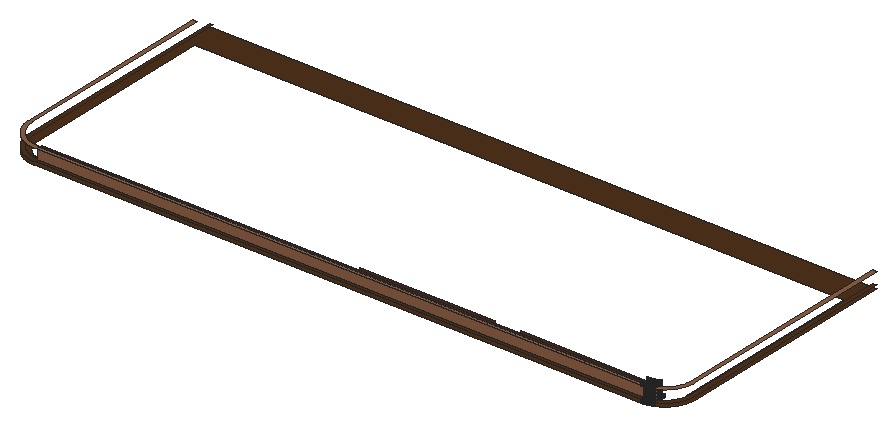
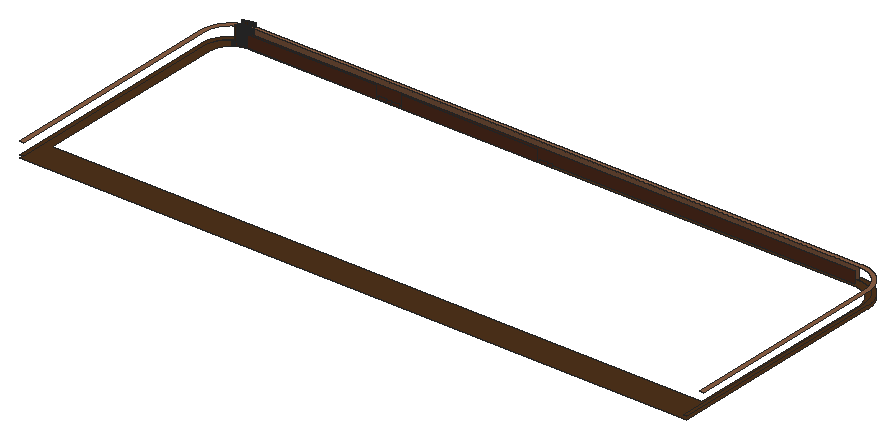
# SketchUp Ruby script. Lengths in inches.
U = 1.inch
M = Sketchup.active_model
def pt(a) = Geom::Point3d.new(a.map { |v| v * U })
def face(e, loops, mat)
  f = e.add_face(loops[0].map { |a| pt(a) })
  loops[1..].each { |l| e.add_face(l.map { |a| pt(a) }).erase! }
  f.material = f.back_material = mat if mat
  f
end
# faces: each face lists its corners as indices into pts; further lists are holes
def faces(e, pts, list, mat = nil) = list.each { |f| face(e, (f[0].is_a?(Array) ? f : [f]).map { |l| l.map { |i| pts[i] } }, mat) }
# xy, xz, yz: faces in a plane at the given z, y or x. An outline is a flat list of corners, or four numbers for a rectangle; further outlines are holes
def ring(l) = l.size == 4 ? [[l[0], l[1]], [l[2], l[1]], [l[2], l[3]], [l[0], l[3]]] : l.each_slice(2).to_a
def flat(e, list, mat, &to3) = list.each { |f| face(e, (f[0].is_a?(Array) ? f : [f]).map { |l| ring(l).map { |u, v| to3.(u, v) } }, mat) }
def xy(e, z, list, mat = nil) = flat(e, list, mat) { |x, y| [x, y, z] }
def xz(e, y, list, mat = nil) = flat(e, list, mat) { |x, z| [x, y, z] }
def yz(e, x, list, mat = nil) = flat(e, list, mat) { |y, z| [x, y, z] }
def lines(e, pts, list) = list.each { |a, b| e.add_line(pt(pts[a]), pt(pts[b])) }
# prism: a flat outline (further loops are holes) pulled along v
def prism(e, loops, v, mat = nil)
  f = face(e, loops, mat); d = Geom::Vector3d.new(v.map { |x| x * U })
  f.pushpull(f.normal.samedirection?(d) ? d.length : -d.length)
end
def box(e, o, s, mat = nil) = prism(e, [[o, [o[0] + s[0], o[1], o[2]], [o[0] + s[0], o[1] + s[1], o[2]], [o[0], o[1] + s[1], o[2]]]], [0, 0, s[2]], mat)
def at(x, y, z, deg = 0) = Geom::Transformation.translation(pt([x, y, z])) * Geom::Transformation.rotation(ORIGIN, Z_AXIS, deg.degrees)
def axes(o, x, y, z) = Geom::Transformation.new([*x, 0, *y, 0, *z, 0, *pt(o).to_a, 1])
def part(name) = M.definitions.add(name)
# library, detail: a bought-in or finely detailed component or shape, given as its bounding box
def library(name, o, s) = part(name).tap { |d| box(d.entities, o, s) }
def detail(e, o, s) = box(e.add_group.entities, o, s)
def put(e, d, t, mat = nil) = e.add_instance(d, t).tap { |i| i.material = mat if mat }
def group(e, t, mat = nil) = e.add_group.tap { |g| g.transformation = t; g.material = mat if mat }.entities
root = M.entities
M.materials.add("1799 AP 8574 BURNISHED CARAMEL").color = [140, 96, 69]
M.materials.add("1816 AP K197 Dark Kaapi-N").color = [79, 50, 27]
M.materials.add("[Wood Cherry Original]1").color = [93, 50, 33]
xy(root,390,[[[65.76,78,65.53,78.01,65.29,78.01,65.06,78.02,64.82,78.04,64.59,78.06,64.35,78.08,64.12,78.1,63.88,78.125,63.65,78.15,63.42,78.1875,63.18,78.22,62.72,78.3,62.49,78.35,62.26,78.39,62.03,78.44,61.8,78.5,61.57,78.55,61.34,78.61,61.11,78.68,60.89,78.74,60.66,78.81,60.4375,78.88,60.21,78.96,59.99,79.03,59.77,79.11,59.55,79.2,59.33,79.28,58.89,79.46,58.68,79.56,58.46,79.65,58.25,79.75,58.04,79.86,57.83,79.96,57.41,80.18,57.2,80.3,57,80.41,56.6,80.65,56.39,80.78,56.2,80.9,56,81.03,55.8,81.17,55.61,81.3,55.42,81.4375,55.23,81.58,55.04,81.72,54.86,81.86,54.67,82.01,54.49,82.16,54.31,82.3125,54.13,82.47,53.96,82.625,53.78,82.78,53.61,82.94,53.44,83.11,53.27,83.27,53.11,83.44,52.94,83.61,52.78,83.78,52.625,83.96,52.47,84.13,52.3125,84.31,52.16,84.49,52.01,84.67,51.86,84.86,51.72,85.04,51.58,85.23,51.4375,85.42,51.3,85.61,51.17,85.8,51.03,86,50.9,86.2,50.78,86.39,50.65,86.6,50.41,87,50.3,87.2,50.18,87.41,49.96,87.83,49.86,88.04,49.75,88.25,49.65,88.46,49.56,88.68,49.46,88.89,49.28,89.33,49.2,89.55,49.11,89.77,49.03,89.99,48.96,90.21,48.88,90.4375,48.81,90.66,48.74,90.89,48.68,91.11,48.61,91.34,48.55,91.57,48.5,91.8,48.44,92.03,48.39,92.26,48.35,92.49,48.3,92.72,48.22,93.18,48.1875,93.42,48.15,93.65,48.125,93.88,48.1,94.12,48.08,94.35,48.06,94.59,48.04,94.82,48.02,95.06,48.01,95.29,48.01,95.53,48,95.76,48,228,438,228,438,95.76,437.99,95.53,437.99,95.29,437.98,95.06,437.96,94.82,437.94,94.59,437.92,94.35,437.9,94.12,437.875,93.88,437.85,93.65,437.8125,93.42,437.78,93.18,437.7,92.72,437.65,92.49,437.61,92.26,437.56,92.03,437.5,91.8,437.45,91.57,437.39,91.34,437.32,91.11,437.26,90.89,437.19,90.66,437.12,90.4375,437.04,90.21,436.97,89.99,436.89,89.77,436.8,89.55,436.72,89.33,436.54,88.89,436.44,88.68,436.35,88.46,436.25,88.25,436.14,88.04,436.04,87.83,435.82,87.41,435.7,87.2,435.59,87,435.35,86.6,435.22,86.39,435.1,86.2,434.97,86,434.83,85.8,434.7,85.61,434.5625,85.42,434.42,85.23,434.28,85.04,434.14,84.86,433.99,84.67,433.84,84.49,433.6875,84.31,433.53,84.13,433.375,83.96,433.22,83.78,433.06,83.61,432.89,83.44,432.73,83.27,432.56,83.11,432.39,82.94,432.22,82.78,432.04,82.625,431.87,82.47,431.69,82.3125,431.51,82.16,431.33,82.01,431.14,81.86,430.96,81.72,430.77,81.58,430.58,81.4375,430.39,81.3,430.2,81.17,430,81.03,429.8,80.9,429.61,80.78,429.4,80.65,429,80.41,428.8,80.3,428.59,80.18,428.17,79.96,427.96,79.86,427.75,79.75,427.54,79.65,427.32,79.56,427.11,79.46,426.67,79.28,426.45,79.2,426.23,79.11,426.01,79.03,425.79,78.96,425.5625,78.88,425.34,78.81,425.11,78.74,424.89,78.68,424.66,78.61,424.43,78.55,424.2,78.5,423.97,78.44,423.74,78.39,423.51,78.35,423.28,78.3,422.82,78.22,422.58,78.1875,422.35,78.15,422.12,78.125,421.88,78.1,421.65,78.08,421.41,78.06,421.18,78.04,420.94,78.02,420.71,78.01,420.47,78.01,420.24,78],[65.66,83,420.34,83,421.19,83.05,421.87,83.13,422.03,83.16,422.2,83.1875,422.37,83.22,422.54,83.25,422.7,83.28,422.87,83.32,423.03,83.36,423.2,83.4,423.36,83.44,423.53,83.49,423.69,83.54,423.86,83.58,424.02,83.64,424.18,83.69,424.34,83.75,424.5,83.8,424.66,83.86,424.82,83.93,424.97,83.99,425.13,84.06,425.29,84.125,425.44,84.19,425.6,84.27,425.75,84.34,426.5,84.74,426.65,84.83,426.79,84.92,426.9375,85.01,427.08,85.1,427.22,85.19,427.36,85.29,427.5,85.38,427.78,85.58,427.91,85.6875,428.05,85.79,428.18,85.9,428.3125,86.01,428.44,86.11,428.57,86.23,428.7,86.34,428.82,86.45,428.95,86.57,429.07,86.6875,429.19,86.81,429.3125,86.93,429.43,87.05,429.55,87.18,429.66,87.3,429.77,87.43,429.89,87.56,429.99,87.6875,430.1,87.82,430.21,87.95,430.3125,88.09,430.42,88.22,430.62,88.5,430.71,88.64,430.81,88.78,430.9,88.92,430.99,89.0625,431.08,89.21,431.17,89.35,431.26,89.5,431.66,90.25,431.73,90.4,431.81,90.56,431.875,90.71,431.94,90.87,432.01,91.03,432.07,91.18,432.14,91.34,432.2,91.5,432.25,91.66,432.31,91.82,432.36,91.98,432.42,92.14,432.46,92.31,432.51,92.47,432.56,92.64,432.6,92.8,432.64,92.97,432.68,93.13,432.72,93.3,432.75,93.46,432.78,93.63,432.8125,93.8,432.84,93.97,432.87,94.13,432.95,94.81,433,95.66,433,211,53,211,53,95.66,53.05,94.81,53.13,94.13,53.16,93.97,53.1875,93.8,53.22,93.63,53.25,93.46,53.28,93.3,53.32,93.13,53.36,92.97,53.4,92.8,53.44,92.64,53.49,92.47,53.54,92.31,53.58,92.14,53.64,91.98,53.69,91.82,53.75,91.66,53.8,91.5,53.86,91.34,53.93,91.18,53.99,91.03,54.06,90.87,54.125,90.71,54.19,90.56,54.27,90.4,54.34,90.25,54.74,89.5,54.83,89.35,54.92,89.21,55.01,89.0625,55.1,88.92,55.19,88.78,55.29,88.64,55.38,88.5,55.58,88.22,55.6875,88.09,55.79,87.95,55.9,87.82,56.01,87.6875,56.11,87.56,56.23,87.43,56.34,87.3,56.45,87.18,56.57,87.05,56.6875,86.93,56.81,86.81,56.93,86.6875,57.05,86.57,57.18,86.45,57.3,86.34,57.43,86.23,57.56,86.11,57.6875,86.01,57.82,85.9,57.95,85.79,58.09,85.6875,58.22,85.58,58.5,85.38,58.64,85.29,58.78,85.19,58.92,85.1,59.0625,85.01,59.21,84.92,59.35,84.83,59.5,84.74,60.25,84.34,60.4,84.27,60.56,84.19,60.71,84.125,60.87,84.06,61.03,83.99,61.18,83.93,61.34,83.86,61.5,83.8,61.66,83.75,61.82,83.69,61.98,83.64,62.14,83.58,62.31,83.54,62.47,83.49,62.64,83.44,62.8,83.4,62.97,83.36,63.13,83.32,63.3,83.28,63.46,83.25,63.63,83.22,63.8,83.1875,63.97,83.16,64.13,83.13,64.81,83.05]]],"1816 AP K197 Dark Kaapi-N")
xy(root,391,[[421.5,84.6,421.92,84.66,421.8,84.64],[421.92,84.66,422.37,84.75,422.8,84.85,423.24,84.97,423.67,85.11,424.09,85.26,424.51,85.43,424.92,85.61,425.32,85.81,425.48,85.9,425.48,85.89,425.35,85.82,425.09,85.6875,424.95,85.62,424.68,85.49,424.4,85.375,423.98,85.21,423.7,85.11,423.12,84.93,422.83,84.85,422.54,84.78,422.24,84.72,422.1,84.69]],"[Wood Cherry Original]1")
xy(root,392,[[65.76,78,420.24,78,420.47,78.01,420.71,78.01,420.94,78.02,421.18,78.04,421.41,78.06,421.65,78.08,421.88,78.1,422.12,78.125,422.35,78.15,422.58,78.1875,422.82,78.22,423.28,78.3,423.51,78.35,423.74,78.39,423.97,78.44,424.2,78.5,424.43,78.55,424.66,78.61,424.89,78.68,425.11,78.74,425.34,78.81,425.5625,78.88,425.79,78.96,426.01,79.03,426.23,79.11,426.45,79.2,426.67,79.28,427.11,79.46,427.32,79.56,427.54,79.65,427.75,79.75,427.96,79.86,428.17,79.96,428.59,80.18,428.8,80.3,429,80.41,429.4,80.65,429.61,80.78,429.8,80.9,430,81.03,430.2,81.17,430.39,81.3,430.58,81.4375,430.77,81.58,430.96,81.72,431.14,81.86,431.33,82.01,431.51,82.16,431.69,82.3125,431.87,82.47,432.04,82.625,432.22,82.78,432.39,82.94,432.56,83.11,432.73,83.27,432.89,83.44,433.06,83.61,433.22,83.78,433.375,83.96,433.53,84.13,433.6875,84.31,433.84,84.49,433.99,84.67,434.14,84.86,434.28,85.04,434.42,85.23,434.5625,85.42,434.7,85.61,434.83,85.8,434.97,86,435.1,86.2,435.22,86.39,435.35,86.6,435.59,87,435.7,87.2,435.82,87.41,436.04,87.83,436.14,88.04,436.25,88.25,436.35,88.46,436.44,88.68,436.54,88.89,436.72,89.33,436.8,89.55,436.89,89.77,436.97,89.99,437.04,90.21,437.12,90.4375,437.19,90.66,437.26,90.89,437.32,91.11,437.39,91.34,437.45,91.57,437.5,91.8,437.56,92.03,437.61,92.26,437.65,92.49,437.7,92.72,437.78,93.18,437.8125,93.42,437.85,93.65,437.875,93.88,437.9,94.12,437.92,94.35,437.94,94.59,437.96,94.82,437.98,95.06,437.99,95.29,437.99,95.53,438,95.76,438,228,436,228,436,95.79,435.99,95.58,435.99,95.37,435.97,94.95,435.95,94.74,435.93,94.54,435.89,94.12,435.83,93.7,435.8,93.5,435.77,93.29,435.73,93.08,435.69,92.88,435.65,92.67,435.61,92.47,435.56,92.26,435.51,92.0625,435.45,91.86,435.4,91.66,435.22,91.06,435.01,90.46,434.9375,90.27,434.86,90.07,434.78,89.88,434.7,89.68,434.62,89.49,434.35,88.92,434.26,88.74,434.16,88.55,434.0625,88.37,433.96,88.18,433.86,88,433.53,87.46,433.42,87.29,433.3,87.11,433.1875,86.9375,433.07,86.77,432.94,86.6,432.82,86.43,432.69,86.26,432.57,86.09,432.43,85.93,432.17,85.61,431.89,85.29,431.61,84.99,431.46,84.84,431.3125,84.6875,431.16,84.54,431.01,84.39,430.71,84.11,430.39,83.83,430.07,83.57,429.91,83.43,429.74,83.31,429.57,83.18,429.4,83.06,429.23,82.93,429.0625,82.8125,428.89,82.7,428.71,82.58,428.54,82.47,428,82.14,427.82,82.04,427.63,81.9375,427.45,81.84,427.26,81.74,427.08,81.65,426.51,81.38,426.32,81.3,426.12,81.22,425.93,81.14,425.73,81.0625,425.54,80.99,424.94,80.78,424.34,80.6,424.14,80.55,423.9375,80.49,423.74,80.44,423.53,80.39,423.33,80.35,423.12,80.31,422.92,80.27,422.71,80.23,422.5,80.2,422.3,80.17,421.88,80.11,421.46,80.07,421.26,80.05,421.05,80.03,420.63,80.01,420.42,80.01,420.21,80,65.79,80,65.58,80.01,65.37,80.01,64.95,80.03,64.74,80.05,64.54,80.07,64.12,80.11,63.7,80.17,63.5,80.2,63.29,80.23,63.08,80.27,62.88,80.31,62.67,80.35,62.47,80.39,62.26,80.44,62.0625,80.49,61.86,80.55,61.66,80.6,61.06,80.78,60.46,80.99,60.27,81.0625,60.07,81.14,59.88,81.22,59.68,81.3,59.49,81.38,58.92,81.65,58.74,81.74,58.55,81.84,58.37,81.9375,58.18,82.04,58,82.14,57.46,82.47,57.29,82.58,57.11,82.7,56.9375,82.8125,56.77,82.93,56.6,83.06,56.43,83.18,56.26,83.31,56.09,83.43,55.93,83.57,55.61,83.83,55.29,84.11,54.99,84.39,54.84,84.54,54.6875,84.6875,54.54,84.84,54.39,84.99,54.11,85.29,53.83,85.61,53.57,85.93,53.43,86.09,53.31,86.26,53.18,86.43,53.06,86.6,52.93,86.77,52.8125,86.9375,52.7,87.11,52.58,87.29,52.47,87.46,52.14,88,52.04,88.18,51.9375,88.37,51.84,88.55,51.74,88.74,51.65,88.92,51.38,89.49,51.3,89.68,51.22,89.88,51.14,90.07,51.0625,90.27,50.99,90.46,50.78,91.06,50.6,91.66,50.55,91.86,50.49,92.0625,50.44,92.26,50.39,92.47,50.35,92.67,50.31,92.88,50.27,93.08,50.23,93.29,50.2,93.5,50.17,93.7,50.11,94.12,50.07,94.54,50.05,94.74,50.03,94.95,50.01,95.37,50.01,95.58,50,95.79,50,228,48,228,48,95.76,48.01,95.53,48.01,95.29,48.02,95.06,48.04,94.82,48.06,94.59,48.08,94.35,48.1,94.12,48.125,93.88,48.15,93.65,48.1875,93.42,48.22,93.18,48.3,92.72,48.35,92.49,48.39,92.26,48.44,92.03,48.5,91.8,48.55,91.57,48.61,91.34,48.68,91.11,48.74,90.89,48.81,90.66,48.88,90.4375,48.96,90.21,49.03,89.99,49.11,89.77,49.2,89.55,49.28,89.33,49.46,88.89,49.56,88.68,49.65,88.46,49.75,88.25,49.86,88.04,49.96,87.83,50.18,87.41,50.3,87.2,50.41,87,50.65,86.6,50.78,86.39,50.9,86.2,51.03,86,51.17,85.8,51.3,85.61,51.4375,85.42,51.58,85.23,51.72,85.04,51.86,84.86,52.01,84.67,52.16,84.49,52.3125,84.31,52.47,84.13,52.625,83.96,52.78,83.78,52.94,83.61,53.11,83.44,53.27,83.27,53.44,83.11,53.61,82.94,53.78,82.78,53.96,82.625,54.13,82.47,54.31,82.3125,54.49,82.16,54.67,82.01,54.86,81.86,55.04,81.72,55.23,81.58,55.42,81.4375,55.61,81.3,55.8,81.17,56,81.03,56.2,80.9,56.39,80.78,56.6,80.65,57,80.41,57.2,80.3,57.41,80.18,57.83,79.96,58.04,79.86,58.25,79.75,58.46,79.65,58.68,79.56,58.89,79.46,59.33,79.28,59.55,79.2,59.77,79.11,59.99,79.03,60.21,78.96,60.4375,78.88,60.66,78.81,60.89,78.74,61.11,78.68,61.34,78.61,61.57,78.55,61.8,78.5,62.03,78.44,62.26,78.39,62.49,78.35,62.72,78.3,63.18,78.22,63.42,78.1875,63.65,78.15,63.88,78.125,64.12,78.1,64.35,78.08,64.59,78.06,64.82,78.04,65.06,78.02,65.29,78.01,65.53,78.01]],"1816 AP K197 Dark Kaapi-N")
xy(root,399,[[65.76,78,65.53,78.01,65.29,78.01,65.06,78.02,64.82,78.04,64.59,78.06,64.35,78.08,64.12,78.1,63.88,78.125,63.65,78.15,63.42,78.1875,63.18,78.22,62.72,78.3,62.49,78.35,62.26,78.39,62.03,78.44,61.8,78.5,61.57,78.55,61.34,78.61,61.11,78.68,60.89,78.74,60.66,78.81,60.4375,78.88,60.21,78.96,59.99,79.03,59.77,79.11,59.55,79.2,59.33,79.28,58.89,79.46,58.68,79.56,58.46,79.65,58.25,79.75,58.04,79.86,57.83,79.96,57.41,80.18,57.2,80.3,57,80.41,56.6,80.65,56.39,80.78,56.2,80.9,56,81.03,55.8,81.17,55.61,81.3,55.42,81.4375,55.23,81.58,55.04,81.72,54.86,81.86,54.67,82.01,54.49,82.16,54.31,82.3125,54.13,82.47,53.96,82.625,53.78,82.78,53.61,82.94,53.44,83.11,53.27,83.27,53.11,83.44,52.94,83.61,52.78,83.78,52.625,83.96,52.47,84.13,52.3125,84.31,52.16,84.49,52.01,84.67,51.86,84.86,51.72,85.04,51.58,85.23,51.4375,85.42,51.3,85.61,51.17,85.8,51.03,86,50.9,86.2,50.78,86.39,50.65,86.6,50.41,87,50.3,87.2,50.18,87.41,49.96,87.83,49.86,88.04,49.75,88.25,49.65,88.46,49.56,88.68,49.46,88.89,49.28,89.33,49.2,89.55,49.11,89.77,49.03,89.99,48.96,90.21,48.88,90.4375,48.81,90.66,48.74,90.89,48.68,91.11,48.61,91.34,48.55,91.57,48.5,91.8,48.44,92.03,48.39,92.26,48.35,92.49,48.3,92.72,48.22,93.18,48.1875,93.42,48.15,93.65,48.125,93.88,48.1,94.12,48.08,94.35,48.06,94.59,48.04,94.82,48.02,95.06,48.01,95.29,48.01,95.53,48,95.76,48,216,50,216,50,95.79,50.01,95.58,50.01,95.37,50.03,94.95,50.05,94.74,50.07,94.54,50.11,94.12,50.17,93.7,50.2,93.5,50.23,93.29,50.27,93.08,50.31,92.88,50.35,92.67,50.39,92.47,50.44,92.26,50.49,92.0625,50.55,91.86,50.6,91.66,50.78,91.06,50.99,90.46,51.0625,90.27,51.14,90.07,51.22,89.88,51.3,89.68,51.38,89.49,51.65,88.92,51.74,88.74,51.84,88.55,51.9375,88.37,52.04,88.18,52.14,88,52.47,87.46,52.58,87.29,52.7,87.11,52.8125,86.9375,52.93,86.77,53.06,86.6,53.18,86.43,53.31,86.26,53.43,86.09,53.57,85.93,53.83,85.61,54.11,85.29,54.39,84.99,54.54,84.84,54.6875,84.6875,54.84,84.54,54.99,84.39,55.29,84.11,55.61,83.83,55.93,83.57,56.09,83.43,56.26,83.31,56.43,83.18,56.6,83.06,56.77,82.93,56.9375,82.8125,57.11,82.7,57.29,82.58,57.46,82.47,58,82.14,58.18,82.04,58.37,81.9375,58.55,81.84,58.74,81.74,58.92,81.65,59.49,81.38,59.68,81.3,59.88,81.22,60.07,81.14,60.27,81.0625,60.46,80.99,61.06,80.78,61.66,80.6,61.86,80.55,62.0625,80.49,62.26,80.44,62.47,80.39,62.67,80.35,62.88,80.31,63.08,80.27,63.29,80.23,63.5,80.2,63.7,80.17,64.12,80.11,64.54,80.07,64.74,80.05,64.95,80.03,65.37,80.01,65.58,80.01,65.79,80,420.21,80,420.42,80.01,420.63,80.01,421.05,80.03,421.26,80.05,421.46,80.07,421.88,80.11,422.3,80.17,422.5,80.2,422.71,80.23,422.92,80.27,423.12,80.31,423.33,80.35,423.53,80.39,423.74,80.44,423.9375,80.49,424.14,80.55,424.34,80.6,424.94,80.78,425.54,80.99,425.73,81.0625,425.93,81.14,426.12,81.22,426.32,81.3,426.51,81.38,427.08,81.65,427.26,81.74,427.45,81.84,427.63,81.9375,427.82,82.04,428,82.14,428.54,82.47,428.71,82.58,428.89,82.7,429.0625,82.8125,429.23,82.93,429.4,83.06,429.57,83.18,429.74,83.31,429.91,83.43,430.07,83.57,430.39,83.83,430.71,84.11,431.01,84.39,431.16,84.54,431.3125,84.6875,431.46,84.84,431.61,84.99,431.89,85.29,432.17,85.61,432.43,85.93,432.57,86.09,432.69,86.26,432.82,86.43,432.94,86.6,433.07,86.77,433.1875,86.9375,433.3,87.11,433.42,87.29,433.53,87.46,433.86,88,433.96,88.18,434.0625,88.37,434.16,88.55,434.26,88.74,434.35,88.92,434.62,89.49,434.7,89.68,434.78,89.88,434.86,90.07,434.9375,90.27,435.01,90.46,435.22,91.06,435.4,91.66,435.45,91.86,435.51,92.0625,435.56,92.26,435.61,92.47,435.65,92.67,435.69,92.88,435.73,93.08,435.77,93.29,435.8,93.5,435.83,93.7,435.89,94.12,435.93,94.54,435.95,94.74,435.97,94.95,435.99,95.37,435.99,95.58,436,95.79,436,228,438,228,438,95.76,437.99,95.53,437.99,95.29,437.98,95.06,437.96,94.82,437.94,94.59,437.92,94.35,437.9,94.12,437.875,93.88,437.85,93.65,437.8125,93.42,437.78,93.18,437.7,92.72,437.65,92.49,437.61,92.26,437.56,92.03,437.5,91.8,437.45,91.57,437.39,91.34,437.32,91.11,437.26,90.89,437.19,90.66,437.12,90.4375,437.04,90.21,436.97,89.99,436.89,89.77,436.8,89.55,436.72,89.33,436.54,88.89,436.44,88.68,436.35,88.46,436.25,88.25,436.14,88.04,436.04,87.83,435.82,87.41,435.7,87.2,435.59,87,435.35,86.6,435.22,86.39,435.1,86.2,434.97,86,434.83,85.8,434.7,85.61,434.5625,85.42,434.42,85.23,434.28,85.04,434.14,84.86,433.99,84.67,433.84,84.49,433.6875,84.31,433.53,84.13,433.375,83.96,433.22,83.78,433.06,83.61,432.89,83.44,432.73,83.27,432.56,83.11,432.39,82.94,432.22,82.78,432.04,82.625,431.87,82.47,431.69,82.3125,431.51,82.16,431.33,82.01,431.14,81.86,430.96,81.72,430.77,81.58,430.58,81.4375,430.39,81.3,430.2,81.17,430,81.03,429.8,80.9,429.61,80.78,429.4,80.65,429,80.41,428.8,80.3,428.59,80.18,428.17,79.96,427.96,79.86,427.75,79.75,427.54,79.65,427.32,79.56,427.11,79.46,426.67,79.28,426.45,79.2,426.23,79.11,426.01,79.03,425.79,78.96,425.5625,78.88,425.34,78.81,425.11,78.74,424.89,78.68,424.66,78.61,424.43,78.55,424.2,78.5,423.97,78.44,423.74,78.39,423.51,78.35,423.28,78.3,422.82,78.22,422.58,78.1875,422.35,78.15,422.12,78.125,421.88,78.1,421.65,78.08,421.41,78.06,421.18,78.04,420.94,78.02,420.71,78.01,420.47,78.01,420.24,78]],"1799 AP 8574 BURNISHED CARAMEL")
xz(root,78,[[420,390,420.24,392],[420,399,420.24,401]],"1816 AP K197 Dark Kaapi-N")
xz(root,78.01,[[420.47,390,420.71,392],[420.47,399,420.71,401]],"1816 AP K197 Dark Kaapi-N")
xz(root,80,[[66.01,392,419.99,399],[419.99,392,420.21,399]],"1799 AP 8574 BURNISHED CARAMEL")
xz(root,80.01,[[420.42,392,420.63,399]],"1799 AP 8574 BURNISHED CARAMEL")
xz(root,83,[[419.98,390,420.17,401],[420.17,390,420.34,401]],"1816 AP K197 Dark Kaapi-N")
xz(root,83,[[66.02,391,419.98,398],[419.98,391,420.17,398],[420.17,391,420.34,398]],"[Wood Cherry Original]1")
xz(root,84.5,[[242,391,244,392.75],[245,391,249,392.75],[250.5,391,329.75,398],[331.25,391,335.25,392.75],[336.25,391,338.25,392.75],
  [339.25,391,343.25,392.75],[344.75,391,419.98,398]],"[Wood Cherry Original]1")
xz(root,84.6,[[421.48,391,421.5,392.75]],"[Wood Cherry Original]1")
p = [[420.24,78,390],[420.47,78.01,390],[420.47,78.01,392],[420.24,78,392],[420.71,78.01,390],[420.94,78.02,390],
  [420.94,78.02,392],[420.71,78.01,392],[421.18,78.04,390],[421.18,78.04,392],[421.41,78.06,390],[421.41,78.06,392],
  [421.65,78.08,390],[421.65,78.08,392],[421.88,78.1,390],[421.88,78.1,392],[422.12,78.125,390],[422.12,78.125,392],
  [422.35,78.15,390],[422.35,78.15,392],[422.58,78.1875,390],[422.58,78.1875,392],[422.82,78.22,390],[422.82,78.22,392],
  [423.05,78.26,390],[423.05,78.26,392],[423.28,78.3,390],[423.28,78.3,392],[423.51,78.35,390],[423.51,78.35,392],
  [423.74,78.39,390],[423.74,78.39,392],[423.97,78.44,390],[423.97,78.44,392],[424.2,78.5,390],[424.2,78.5,392],
  [424.43,78.55,390],[424.43,78.55,392],[424.66,78.61,390],[424.66,78.61,392],[424.89,78.68,390],[424.89,78.68,392],
  [425.11,78.74,390],[425.11,78.74,392],[425.34,78.81,390],[425.34,78.81,392],[425.5625,78.88,390],[425.5625,78.88,392],
  [425.79,78.96,390],[425.79,78.96,392],[426.01,79.03,390],[426.01,79.03,392],[426.23,79.11,390],[426.23,79.11,392],
  [426.45,79.2,390],[426.45,79.2,392],[426.67,79.28,390],[426.67,79.28,392],[426.89,79.37,390],[426.89,79.37,392],
  [427.11,79.46,390],[427.11,79.46,392],[420.34,83,401],[420.51,83.01,401],[420.51,83.01,390],[420.34,83,390],
  [420.68,83.02,401],[420.68,83.02,390],[420.85,83.03,401],[420.85,83.03,390],[421.02,83.04,401],[421.02,83.04,390],
  [421.19,83.05,401],[421.19,83.05,390],[421.36,83.07,401],[421.36,83.07,390],[421.53,83.09,401],[421.53,83.09,390],
  [421.7,83.11,401],[421.7,83.11,390],[421.87,83.13,401],[421.87,83.13,390],[422.03,83.16,401],[422.03,83.16,390],
  [422.2,83.1875,401],[422.2,83.1875,390],[422.37,83.22,401],[422.37,83.22,390],[422.54,83.25,401],[422.54,83.25,390],
  [422.7,83.28,401],[422.7,83.28,390],[422.87,83.32,401],[422.87,83.32,390],[423.03,83.36,401],[423.03,83.36,390],
  [423.2,83.4,401],[423.2,83.4,390],[423.36,83.44,401],[423.36,83.44,390],[423.53,83.49,401],[423.53,83.49,390],
  [423.69,83.54,401],[423.69,83.54,390],[423.86,83.58,401],[423.86,83.58,390],[424.02,83.64,401],[424.02,83.64,390],
  [424.18,83.69,401],[424.18,83.69,390],[424.34,83.75,401],[424.34,83.75,390],[424.5,83.8,401],[424.5,83.8,390],
  [424.66,83.86,401],[424.66,83.86,390],[424.82,83.93,401],[424.82,83.93,390],[424.97,83.99,401],[424.97,83.99,390],
  [425.13,84.06,401],[425.13,84.06,390],[425.29,84.125,401],[425.29,84.125,390],[425.44,84.19,401],[425.44,84.19,390],
  [425.6,84.27,401],[425.6,84.27,390],[425.75,84.34,401],[425.75,84.34,390],[425.9,84.42,401],[425.9,84.42,390],
  [426.05,84.5,401],[426.05,84.5,390],[426.2,84.58,401],[426.2,84.58,390],[426.35,84.66,401],[426.35,84.66,390],
  [426.5,84.74,401],[426.5,84.74,390],[426.65,84.83,401],[426.65,84.83,390],[426.79,84.92,401],[426.79,84.92,390],
  [426.9375,85.01,401],[426.9375,85.01,390],[427.08,85.1,401],[427.08,85.1,390],[420.34,83,391],[420.51,83.01,391],
  [420.51,83.01,398],[420.34,83,398],[420.68,83.02,391],[420.68,83.02,398],[420.85,83.03,391],[420.85,83.03,398],
  [421.02,83.04,391],[421.02,83.04,398],[421.19,83.05,391],[421.19,83.05,398],[421.36,83.07,391],[421.36,83.07,398],
  [421.53,83.09,391],[421.53,83.09,398],[421.7,83.11,391],[421.7,83.11,398],[421.87,83.13,391],[421.87,83.13,398],
  [422.03,83.16,391],[422.03,83.16,398],[422.2,83.1875,391],[422.2,83.1875,398],[422.37,83.22,391],[422.37,83.22,398],
  [422.54,83.25,391],[422.54,83.25,398],[422.7,83.28,391],[422.7,83.28,398],[422.87,83.32,391],[422.87,83.32,398],
  [423.03,83.36,391],[423.03,83.36,398],[423.2,83.4,391],[423.2,83.4,398],[423.36,83.44,391],[423.36,83.44,398],
  [423.53,83.49,391],[423.53,83.49,398],[423.69,83.54,391],[423.69,83.54,398],[423.86,83.58,391],[423.86,83.58,398],
  [424.02,83.64,391],[424.02,83.64,398],[424.18,83.69,391],[424.18,83.69,398],[424.34,83.75,391],[424.34,83.75,398],
  [424.5,83.8,391],[424.5,83.8,398],[424.66,83.86,391],[424.66,83.86,398],[424.82,83.93,391],[424.82,83.93,398],
  [424.97,83.99,391],[424.97,83.99,398],[425.13,84.06,391],[425.13,84.06,398],[425.29,84.125,391],[425.29,84.125,398],
  [425.44,84.19,391],[425.44,84.19,398],[425.6,84.27,391],[425.6,84.27,398],[425.75,84.34,391],[425.75,84.34,398],
  [425.9,84.42,391],[425.9,84.42,398],[426.05,84.5,391],[426.05,84.5,398],[426.2,84.58,391],[426.2,84.58,398],
  [421.92,84.66,391],[421.5,84.6,391],[421.5,84.6,392.75],[421.92,84.66,392.75],[426.35,84.66,391],[426.35,84.66,398],
  [422.37,84.75,391],[422.37,84.75,392.75],[422.8,84.85,391],[422.8,84.85,392.75],[426.48,84.73,391],[426.5,84.74,391],
  [426.5,84.74,398],[426.65,84.83,391],[426.65,84.83,398],[426.79,84.92,391],[426.79,84.92,398],[423.24,84.97,391],
  [423.24,84.97,392.75],[426.9375,85.01,391],[426.9375,85.01,398],[423.67,85.11,391],[423.67,85.11,392.75],[427.08,85.1,391],
  [427.08,85.1,398],[424.09,85.26,391],[424.09,85.26,392.75],[424.51,85.43,391],[424.51,85.43,392.75],[424.92,85.61,391],
  [424.92,85.61,392.75],[425.32,85.81,391],[425.32,85.81,392.75],[425.48,85.9,391],[425.48,85.9,392.75],[426.51,86.52,391],
  [426.48,86.5,391],[426.48,86.5,392.75],[426.51,86.52,392.75],[426.64,86.61,391],[426.64,86.61,392.75],[426.88,86.79,391],
  [426.88,86.79,392.75],[427.12,86.97,391],[427.12,86.97,392.75],[420.21,80,392],[420.42,80.01,392],[420.42,80.01,399],
  [420.21,80,399],[420.63,80.01,392],[420.84,80.02,392],[420.84,80.02,399],[420.63,80.01,399],[421.05,80.03,392],
  [421.05,80.03,399],[421.26,80.05,392],[421.26,80.05,399],[421.46,80.07,392],[421.46,80.07,399],[421.67,80.09,392],
  [421.67,80.09,399],[421.88,80.11,392],[421.88,80.11,399],[422.09,80.14,392],[422.09,80.14,399],[422.3,80.17,392],
  [422.3,80.17,399],[422.5,80.2,392],[422.5,80.2,399],[422.71,80.23,392],[422.71,80.23,399],[422.92,80.27,392],
  [422.92,80.27,399],[423.12,80.31,392],[423.12,80.31,399],[423.33,80.35,392],[423.33,80.35,399],[423.53,80.39,392],
  [423.53,80.39,399],[423.74,80.44,392],[423.74,80.44,399],[423.9375,80.49,392],[423.9375,80.49,399],[424.14,80.55,392],
  [424.14,80.55,399],[424.34,80.6,392],[424.34,80.6,399],[424.54,80.66,392],[424.54,80.66,399],[424.74,80.72,392],
  [424.74,80.72,399],[424.94,80.78,392],[424.94,80.78,399],[425.14,80.85,392],[425.14,80.85,399],[425.34,80.92,392],
  [425.34,80.92,399],[425.54,80.99,392],[425.54,80.99,399],[425.73,81.0625,392],[425.73,81.0625,399],[425.93,81.14,392],
  [425.93,81.14,399],[426.12,81.22,392],[426.12,81.22,399],[426.32,81.3,392],[426.32,81.3,399],[426.51,81.38,392],
  [426.51,81.38,399],[426.7,81.47,392],[426.7,81.47,399],[426.89,81.56,392],[426.89,81.56,399],[427.08,81.65,392],
  [427.08,81.65,399],[420.24,78,399],[420.47,78.01,399],[420.47,78.01,401],[420.24,78,401],[420.71,78.01,399],
  [420.94,78.02,399],[420.94,78.02,401],[420.71,78.01,401],[421.18,78.04,399],[421.18,78.04,401],[421.41,78.06,399],
  [421.41,78.06,401],[421.65,78.08,399],[421.65,78.08,401],[421.88,78.1,399],[421.88,78.1,401],[422.12,78.125,399],
  [422.12,78.125,401],[422.35,78.15,399],[422.35,78.15,401],[422.58,78.1875,399],[422.58,78.1875,401],[422.82,78.22,399],
  [422.82,78.22,401],[423.05,78.26,399],[423.05,78.26,401],[423.28,78.3,399],[423.28,78.3,401],[423.51,78.35,399],
  [423.51,78.35,401],[423.74,78.39,399],[423.74,78.39,401],[423.97,78.44,399],[423.97,78.44,401],[424.2,78.5,399],
  [424.2,78.5,401],[424.43,78.55,399],[424.43,78.55,401],[424.66,78.61,399],[424.66,78.61,401],[424.89,78.68,399],
  [424.89,78.68,401],[425.11,78.74,399],[425.11,78.74,401],[425.34,78.81,399],[425.34,78.81,401],[425.5625,78.88,399],
  [425.5625,78.88,401],[425.79,78.96,399],[425.79,78.96,401],[426.01,79.03,399],[426.01,79.03,401],[426.23,79.11,399],
  [426.23,79.11,401],[426.45,79.2,399],[426.45,79.2,401],[426.67,79.28,399],[426.67,79.28,401],[426.89,79.37,399],
  [426.89,79.37,401],[427.11,79.46,399],[427.11,79.46,401],[426.48,84.5,391]]
faces(root,p,[[0,1,2,3],[4,5,6,7],[5,8,9,6],[8,10,11,9],[10,12,13,11],[12,14,15,13],[14,16,17,15],[16,18,19,17],
  [18,20,21,19],[20,22,23,21],[22,24,25,23],[24,26,27,25],[26,28,29,27],[28,30,31,29],[30,32,33,31],[32,34,35,33],
  [34,36,37,35],[36,38,39,37],[38,40,41,39],[40,42,43,41],[42,44,45,43],[44,46,47,45],[46,48,49,47],[48,50,51,49],
  [50,52,53,51],[52,54,55,53],[54,56,57,55],[56,58,59,57],[58,60,61,59],[62,63,64,65],[63,66,67,64],[66,68,69,67],
  [68,70,71,69],[70,72,73,71],[72,74,75,73],[74,76,77,75],[76,78,79,77],[78,80,81,79],[80,82,83,81],[82,84,85,83],
  [84,86,87,85],[86,88,89,87],[88,90,91,89],[90,92,93,91],[92,94,95,93],[94,96,97,95],[96,98,99,97],[98,100,101,99],
  [100,102,103,101],[102,104,105,103],[104,106,107,105],[106,108,109,107],[108,110,111,109],[110,112,113,111],[112,114,115,113],[114,116,117,115],
  [116,118,119,117],[118,120,121,119],[120,122,123,121],[122,124,125,123],[124,126,127,125],[126,128,129,127],[128,130,131,129],[130,132,133,131],
  [132,134,135,133],[134,136,137,135],[136,138,139,137],[138,140,141,139],[140,142,143,141],[142,144,145,143],[144,146,147,145],[337,338,339,340],
  [341,342,343,344],[342,345,346,343],[345,347,348,346],[347,349,350,348],[349,351,352,350],[351,353,354,352],[353,355,356,354],[355,357,358,356],
  [357,359,360,358],[359,361,362,360],[361,363,364,362],[363,365,366,364],[365,367,368,366],[367,369,370,368],[369,371,372,370],[371,373,374,372],
  [373,375,376,374],[375,377,378,376],[377,379,380,378],[379,381,382,380],[381,383,384,382],[383,385,386,384],[385,387,388,386],[387,389,390,388],
  [389,391,392,390],[391,393,394,392],[393,395,396,394],[395,397,398,396]],"1816 AP K197 Dark Kaapi-N")
faces(root,p,[[148,149,150,151],[149,152,153,150],[152,154,155,153],[154,156,157,155],[156,158,159,157],[158,160,161,159],[160,162,163,161],[162,164,165,163],
  [164,166,167,165],[166,168,169,167],[168,170,171,169],[170,172,173,171],[172,174,175,173],[174,176,177,175],[176,178,179,177],[178,180,181,179],
  [180,182,183,181],[182,184,185,183],[184,186,187,185],[186,188,189,187],[188,190,191,189],[190,192,193,191],[192,194,195,193],[194,196,197,195],
  [196,198,199,197],[198,200,201,199],[200,202,203,201],[202,204,205,203],[204,206,207,205],[206,208,209,207],[208,210,211,209],[210,212,213,211],
  [212,214,215,213],[214,216,217,215],[216,218,219,217],[218,220,221,219],[222,223,224,225],[220,226,227,221],[228,222,225,229],[230,228,229,231],
  [226,232,233,234,227],[233,235,236,234],[235,237,238,236],[239,230,231,240],[237,241,242,238],[243,239,240,244],[241,245,246,242],[247,243,244,248],
  [249,247,248,250],[251,249,250,252],[253,251,252,254],[255,253,254,256],[257,258,259,260],[261,257,260,262],[263,261,262,264],[265,263,264,266]],"[Wood Cherry Original]1")
faces(root,p,[[267,268,269,270],[271,272,273,274],[272,275,276,273],[275,277,278,276],[277,279,280,278],[279,281,282,280],[281,283,284,282],[283,285,286,284],
  [285,287,288,286],[287,289,290,288],[289,291,292,290],[291,293,294,292],[293,295,296,294],[295,297,298,296],[297,299,300,298],[299,301,302,300],
  [301,303,304,302],[303,305,306,304],[305,307,308,306],[307,309,310,308],[309,311,312,310],[311,313,314,312],[313,315,316,314],[315,317,318,316],
  [317,319,320,318],[319,321,322,320],[321,323,324,322],[323,325,326,324],[325,327,328,326],[327,329,330,328],[329,331,332,330],[331,333,334,332],
  [333,335,336,334]],"1799 AP 8574 BURNISHED CARAMEL")
lines(root,p,[[232,399]])
